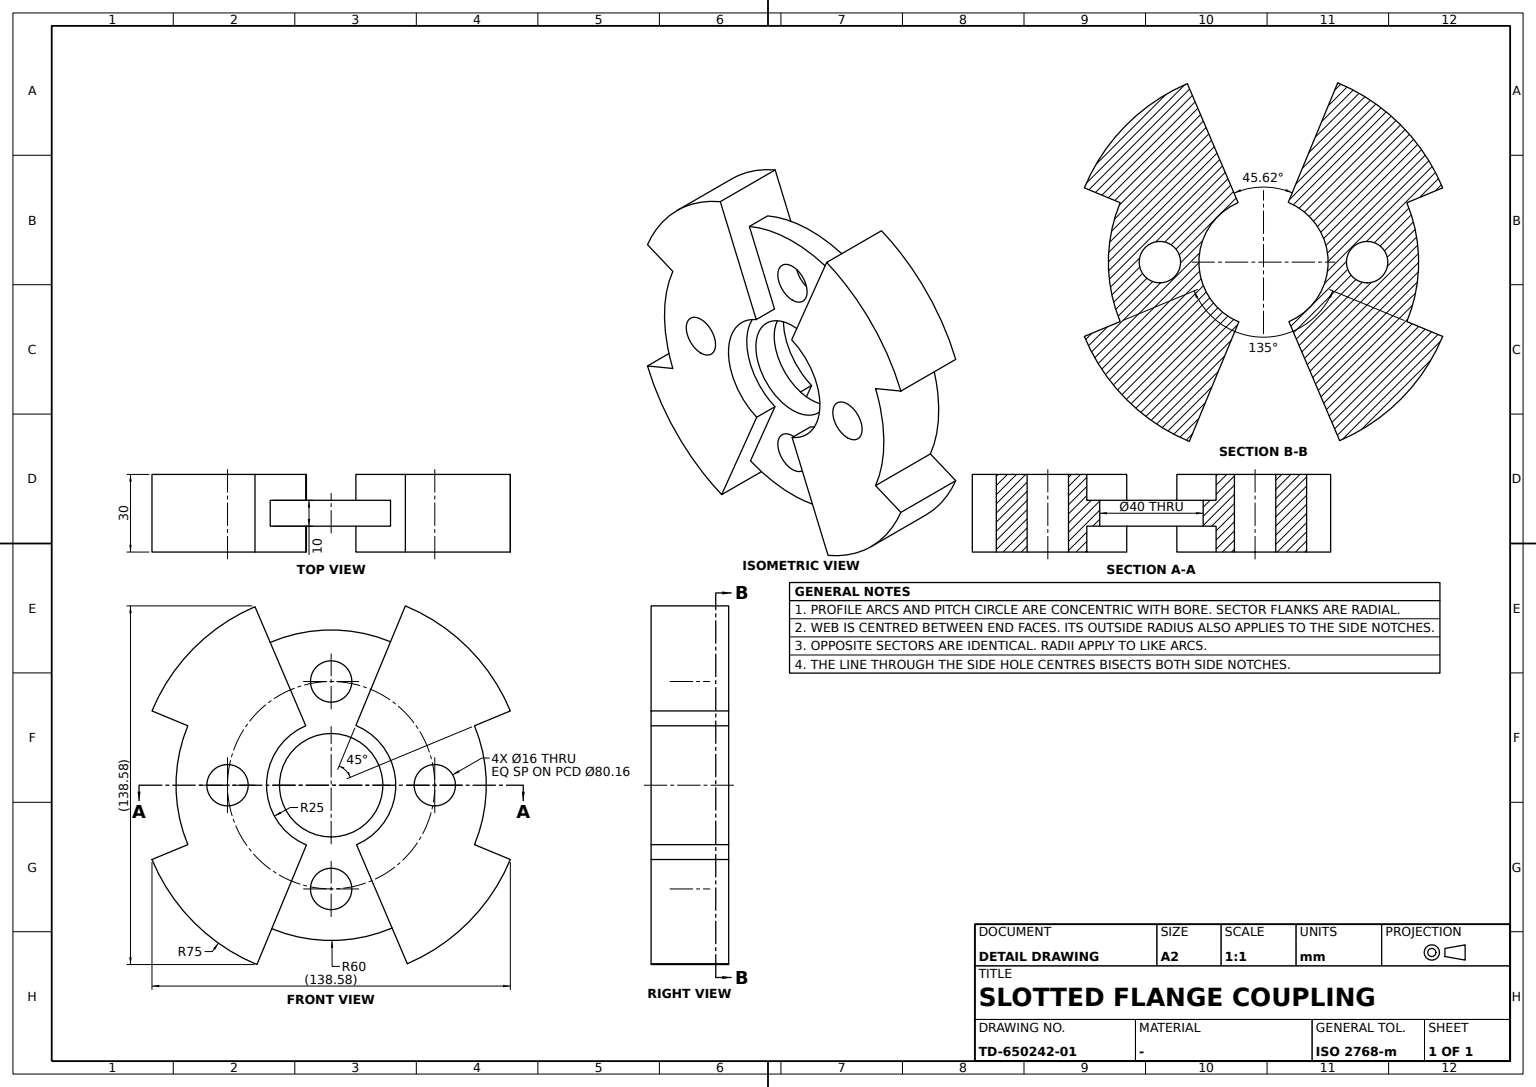
ISO-10303-21;
HEADER;
FILE_DESCRIPTION((''),'2;1');
FILE_NAME('','',(''),(''),'','','');
FILE_SCHEMA(('AUTOMOTIVE_DESIGN'));
ENDSEC;
DATA;
#1=APPLICATION_CONTEXT('');
#2=PRODUCT_CONTEXT('',#1,'mechanical');
#3=PRODUCT('','','',(#2));
#4=PRODUCT_DEFINITION_FORMATION('','',#3);
#5=PRODUCT_DEFINITION_CONTEXT('',#1,'design');
#6=PRODUCT_DEFINITION('','',#4,#5);
#7=PRODUCT_DEFINITION_SHAPE('','',#6);
#8=(LENGTH_UNIT()NAMED_UNIT(*)SI_UNIT(.MILLI.,.METRE.));
#9=(NAMED_UNIT(*)PLANE_ANGLE_UNIT()SI_UNIT($,.RADIAN.));
#10=(NAMED_UNIT(*)SI_UNIT($,.STERADIAN.)SOLID_ANGLE_UNIT());
#11=UNCERTAINTY_MEASURE_WITH_UNIT(LENGTH_MEASURE(0.005),#8,'distance_accuracy_value','');
#12=(GEOMETRIC_REPRESENTATION_CONTEXT(3)GLOBAL_UNCERTAINTY_ASSIGNED_CONTEXT((#11))GLOBAL_UNIT_ASSIGNED_CONTEXT((#8,#9,#10))REPRESENTATION_CONTEXT('',''));
#13=CARTESIAN_POINT('',(-5.,0.,-20.));
#14=VERTEX_POINT('',#13);
#15=CARTESIAN_POINT('',(-5.,0.,0.));
#16=DIRECTION('',(1.,0.,0.));
#17=DIRECTION('',(0.,0.,-1.));
#18=AXIS2_PLACEMENT_3D('',#15,#16,#17);
#19=CIRCLE('',#18,20.);
#20=EDGE_CURVE('',#14,#14,#19,.T.);
#21=ORIENTED_EDGE('',*,*,#20,.F.);
#22=EDGE_LOOP('',(#21));
#23=FACE_BOUND('',#22,.T.);
#24=CARTESIAN_POINT('',(5.,0.,-20.));
#25=VERTEX_POINT('',#24);
#26=CARTESIAN_POINT('',(5.,0.,0.));
#27=AXIS2_PLACEMENT_3D('',#26,#16,#17);
#28=CIRCLE('',#27,20.);
#29=EDGE_CURVE('',#25,#25,#28,.T.);
#30=ORIENTED_EDGE('',*,*,#29,.T.);
#31=EDGE_LOOP('',(#30));
#32=FACE_BOUND('',#31,.T.);
#33=CARTESIAN_POINT('',(0.,0.,0.));
#34=DIRECTION('',(0.,1.,0.));
#35=AXIS2_PLACEMENT_3D('',#33,#16,#34);
#36=CYLINDRICAL_SURFACE('',#35,20.);
#37=ADVANCED_FACE('',(#23,#32),#36,.F.);
#38=CARTESIAN_POINT('',(15.,-69.290965,-28.701257));
#39=VERTEX_POINT('',#38);
#40=CARTESIAN_POINT('',(15.,-28.701257,-69.290965));
#41=VERTEX_POINT('',#40);
#42=CARTESIAN_POINT('',(15.,0.,0.));
#43=AXIS2_PLACEMENT_3D('',#42,#16,#17);
#44=CIRCLE('',#43,75.);
#45=EDGE_CURVE('',#39,#41,#44,.T.);
#46=ORIENTED_EDGE('',*,*,#45,.F.);
#47=CARTESIAN_POINT('',(-15.,-69.290965,-28.701257));
#48=VERTEX_POINT('',#47);
#49=VECTOR('',#16,1000.);
#50=LINE('',#47,#49);
#51=EDGE_CURVE('',#48,#39,#50,.T.);
#52=ORIENTED_EDGE('',*,*,#51,.F.);
#53=CARTESIAN_POINT('',(-15.,-28.701257,-69.290965));
#54=VERTEX_POINT('',#53);
#55=CARTESIAN_POINT('',(-15.,0.,0.));
#56=AXIS2_PLACEMENT_3D('',#55,#16,#17);
#57=CIRCLE('',#56,75.);
#58=EDGE_CURVE('',#48,#54,#57,.T.);
#59=ORIENTED_EDGE('',*,*,#58,.T.);
#60=LINE('',#53,#49);
#61=EDGE_CURVE('',#54,#41,#60,.T.);
#62=ORIENTED_EDGE('',*,*,#61,.T.);
#63=EDGE_LOOP('',(#46,#52,#59,#62));
#64=FACE_BOUND('',#63,.T.);
#65=CYLINDRICAL_SURFACE('',#35,75.);
#66=ADVANCED_FACE('',(#64),#65,.T.);
#67=CARTESIAN_POINT('',(-15.,-55.432772,22.961006));
#68=VERTEX_POINT('',#67);
#69=CARTESIAN_POINT('',(-15.,-55.432772,-22.961006));
#70=VERTEX_POINT('',#69);
#71=CIRCLE('',#56,60.);
#72=EDGE_CURVE('',#68,#70,#71,.T.);
#73=ORIENTED_EDGE('',*,*,#72,.T.);
#74=CARTESIAN_POINT('',(15.,-55.432772,-22.961006));
#75=VERTEX_POINT('',#74);
#76=LINE('',#69,#49);
#77=EDGE_CURVE('',#70,#75,#76,.T.);
#78=ORIENTED_EDGE('',*,*,#77,.T.);
#79=CARTESIAN_POINT('',(15.,-55.432772,22.961006));
#80=VERTEX_POINT('',#79);
#81=CIRCLE('',#43,60.);
#82=EDGE_CURVE('',#80,#75,#81,.T.);
#83=ORIENTED_EDGE('',*,*,#82,.F.);
#84=LINE('',#67,#49);
#85=EDGE_CURVE('',#68,#80,#84,.T.);
#86=ORIENTED_EDGE('',*,*,#85,.F.);
#87=EDGE_LOOP('',(#73,#78,#83,#86));
#88=FACE_BOUND('',#87,.T.);
#89=CYLINDRICAL_SURFACE('',#35,60.);
#90=ADVANCED_FACE('',(#88),#89,.T.);
#91=CARTESIAN_POINT('',(-15.,-69.290965,28.701257));
#92=VERTEX_POINT('',#91);
#93=DIRECTION('',(0.,0.923879533,-0.382683432));
#94=VECTOR('',#93,1000.);
#95=LINE('',#55,#94);
#96=EDGE_CURVE('',#92,#68,#95,.T.);
#97=ORIENTED_EDGE('',*,*,#96,.T.);
#98=ORIENTED_EDGE('',*,*,#85,.T.);
#99=CARTESIAN_POINT('',(15.,-69.290965,28.701257));
#100=VERTEX_POINT('',#99);
#101=LINE('',#42,#94);
#102=EDGE_CURVE('',#100,#80,#101,.T.);
#103=ORIENTED_EDGE('',*,*,#102,.F.);
#104=LINE('',#91,#49);
#105=EDGE_CURVE('',#92,#100,#104,.T.);
#106=ORIENTED_EDGE('',*,*,#105,.F.);
#107=EDGE_LOOP('',(#97,#98,#103,#106));
#108=FACE_BOUND('',#107,.T.);
#109=CARTESIAN_POINT('',(0.,-69.290965,28.701257));
#110=DIRECTION('',(0.,-0.382683432,-0.923879533));
#111=AXIS2_PLACEMENT_3D('',#109,#110,#93);
#112=PLANE('',#111);
#113=ADVANCED_FACE('',(#108),#112,.T.);
#114=CARTESIAN_POINT('',(5.,-9.818454,22.991258));
#115=VERTEX_POINT('',#114);
#116=CARTESIAN_POINT('',(15.,-9.818454,22.991258));
#117=VERTEX_POINT('',#116);
#118=LINE('',#114,#49);
#119=EDGE_CURVE('',#115,#117,#118,.T.);
#120=ORIENTED_EDGE('',*,*,#119,.T.);
#121=CARTESIAN_POINT('',(15.,-9.567086,-23.096988));
#122=VERTEX_POINT('',#121);
#123=CIRCLE('',#43,25.);
#124=EDGE_CURVE('',#117,#122,#123,.T.);
#125=ORIENTED_EDGE('',*,*,#124,.T.);
#126=CARTESIAN_POINT('',(5.,-9.567086,-23.096988));
#127=VERTEX_POINT('',#126);
#128=LINE('',#126,#49);
#129=EDGE_CURVE('',#127,#122,#128,.T.);
#130=ORIENTED_EDGE('',*,*,#129,.F.);
#131=CIRCLE('',#27,25.);
#132=EDGE_CURVE('',#115,#127,#131,.T.);
#133=ORIENTED_EDGE('',*,*,#132,.F.);
#134=EDGE_LOOP('',(#120,#125,#130,#133));
#135=FACE_BOUND('',#134,.T.);
#136=CYLINDRICAL_SURFACE('',#35,25.);
#137=ADVANCED_FACE('',(#135),#136,.F.);
#138=CARTESIAN_POINT('',(-15.,55.432772,-22.961006));
#139=VERTEX_POINT('',#138);
#140=CARTESIAN_POINT('',(15.,55.432772,-22.961006));
#141=VERTEX_POINT('',#140);
#142=LINE('',#138,#49);
#143=EDGE_CURVE('',#139,#141,#142,.T.);
#144=ORIENTED_EDGE('',*,*,#143,.F.);
#145=CARTESIAN_POINT('',(-15.,55.432772,22.961006));
#146=VERTEX_POINT('',#145);
#147=EDGE_CURVE('',#139,#146,#71,.T.);
#148=ORIENTED_EDGE('',*,*,#147,.T.);
#149=CARTESIAN_POINT('',(15.,55.432772,22.961006));
#150=VERTEX_POINT('',#149);
#151=LINE('',#145,#49);
#152=EDGE_CURVE('',#146,#150,#151,.T.);
#153=ORIENTED_EDGE('',*,*,#152,.T.);
#154=EDGE_CURVE('',#141,#150,#81,.T.);
#155=ORIENTED_EDGE('',*,*,#154,.F.);
#156=EDGE_LOOP('',(#144,#148,#153,#155));
#157=FACE_BOUND('',#156,.T.);
#158=ADVANCED_FACE('',(#157),#89,.T.);
#159=CARTESIAN_POINT('',(15.,-40.077698,-8.));
#160=VERTEX_POINT('',#159);
#161=CARTESIAN_POINT('',(15.,-40.077698,0.));
#162=AXIS2_PLACEMENT_3D('',#161,#16,#17);
#163=CIRCLE('',#162,8.);
#164=EDGE_CURVE('',#160,#160,#163,.T.);
#165=ORIENTED_EDGE('',*,*,#164,.F.);
#166=EDGE_LOOP('',(#165));
#167=FACE_BOUND('',#166,.T.);
#168=DIRECTION('',(0.,0.382683432,0.923879533));
#169=VECTOR('',#168,1000.);
#170=LINE('',#42,#169);
#171=EDGE_CURVE('',#41,#122,#170,.T.);
#172=ORIENTED_EDGE('',*,*,#171,.T.);
#173=ORIENTED_EDGE('',*,*,#124,.F.);
#174=CARTESIAN_POINT('',(15.,-29.455362,68.973775));
#175=VERTEX_POINT('',#174);
#176=DIRECTION('',(0.,-0.392738156,0.919650336));
#177=VECTOR('',#176,1000.);
#178=LINE('',#42,#177);
#179=EDGE_CURVE('',#117,#175,#178,.T.);
#180=ORIENTED_EDGE('',*,*,#179,.T.);
#181=EDGE_CURVE('',#175,#100,#44,.T.);
#182=ORIENTED_EDGE('',*,*,#181,.T.);
#183=ORIENTED_EDGE('',*,*,#102,.T.);
#184=ORIENTED_EDGE('',*,*,#82,.T.);
#185=DIRECTION('',(0.,0.923879533,0.382683432));
#186=VECTOR('',#185,1000.);
#187=LINE('',#42,#186);
#188=EDGE_CURVE('',#39,#75,#187,.T.);
#189=ORIENTED_EDGE('',*,*,#188,.F.);
#190=ORIENTED_EDGE('',*,*,#45,.T.);
#191=EDGE_LOOP('',(#172,#173,#180,#182,#183,#184,#189,#190));
#192=FACE_BOUND('',#191,.T.);
#193=AXIS2_PLACEMENT_3D('',#42,#16,#34);
#194=PLANE('',#193);
#195=ADVANCED_FACE('',(#167,#192),#194,.T.);
#196=CARTESIAN_POINT('',(5.,9.567086,23.096988));
#197=VERTEX_POINT('',#196);
#198=CARTESIAN_POINT('',(15.,9.567086,23.096988));
#199=VERTEX_POINT('',#198);
#200=LINE('',#196,#49);
#201=EDGE_CURVE('',#197,#199,#200,.T.);
#202=ORIENTED_EDGE('',*,*,#201,.F.);
#203=CARTESIAN_POINT('',(5.,9.818454,-22.991258));
#204=VERTEX_POINT('',#203);
#205=EDGE_CURVE('',#204,#197,#131,.T.);
#206=ORIENTED_EDGE('',*,*,#205,.F.);
#207=CARTESIAN_POINT('',(15.,9.818454,-22.991258));
#208=VERTEX_POINT('',#207);
#209=LINE('',#203,#49);
#210=EDGE_CURVE('',#204,#208,#209,.T.);
#211=ORIENTED_EDGE('',*,*,#210,.T.);
#212=EDGE_CURVE('',#208,#199,#123,.T.);
#213=ORIENTED_EDGE('',*,*,#212,.T.);
#214=EDGE_LOOP('',(#202,#206,#211,#213));
#215=FACE_BOUND('',#214,.T.);
#216=ADVANCED_FACE('',(#215),#136,.F.);
#217=ORIENTED_EDGE('',*,*,#143,.T.);
#218=CARTESIAN_POINT('',(15.,69.290965,-28.701257));
#219=VERTEX_POINT('',#218);
#220=EDGE_CURVE('',#141,#219,#101,.T.);
#221=ORIENTED_EDGE('',*,*,#220,.T.);
#222=CARTESIAN_POINT('',(-15.,69.290965,-28.701257));
#223=VERTEX_POINT('',#222);
#224=LINE('',#222,#49);
#225=EDGE_CURVE('',#223,#219,#224,.T.);
#226=ORIENTED_EDGE('',*,*,#225,.F.);
#227=EDGE_CURVE('',#139,#223,#95,.T.);
#228=ORIENTED_EDGE('',*,*,#227,.F.);
#229=EDGE_LOOP('',(#217,#221,#226,#228));
#230=FACE_BOUND('',#229,.T.);
#231=ADVANCED_FACE('',(#230),#112,.F.);
#232=ORIENTED_EDGE('',*,*,#171,.F.);
#233=ORIENTED_EDGE('',*,*,#61,.F.);
#234=CARTESIAN_POINT('',(-15.,-9.567086,-23.096988));
#235=VERTEX_POINT('',#234);
#236=LINE('',#55,#169);
#237=EDGE_CURVE('',#54,#235,#236,.T.);
#238=ORIENTED_EDGE('',*,*,#237,.T.);
#239=CARTESIAN_POINT('',(-5.,-9.567086,-23.096988));
#240=VERTEX_POINT('',#239);
#241=LINE('',#234,#49);
#242=EDGE_CURVE('',#235,#240,#241,.T.);
#243=ORIENTED_EDGE('',*,*,#242,.T.);
#244=CARTESIAN_POINT('',(-5.,-22.961006,-55.432772));
#245=VERTEX_POINT('',#244);
#246=LINE('',#15,#169);
#247=EDGE_CURVE('',#245,#240,#246,.T.);
#248=ORIENTED_EDGE('',*,*,#247,.F.);
#249=CARTESIAN_POINT('',(5.,-22.961006,-55.432772));
#250=VERTEX_POINT('',#249);
#251=LINE('',#244,#49);
#252=EDGE_CURVE('',#245,#250,#251,.T.);
#253=ORIENTED_EDGE('',*,*,#252,.T.);
#254=LINE('',#26,#169);
#255=EDGE_CURVE('',#250,#127,#254,.T.);
#256=ORIENTED_EDGE('',*,*,#255,.T.);
#257=ORIENTED_EDGE('',*,*,#129,.T.);
#258=EDGE_LOOP('',(#232,#233,#238,#243,#248,#253,#256,#257));
#259=FACE_BOUND('',#258,.T.);
#260=CARTESIAN_POINT('',(0.,-28.701257,-69.290965));
#261=AXIS2_PLACEMENT_3D('',#260,#93,#168);
#262=PLANE('',#261);
#263=ADVANCED_FACE('',(#259),#262,.T.);
#264=CARTESIAN_POINT('',(-15.,9.567086,23.096988));
#265=VERTEX_POINT('',#264);
#266=CARTESIAN_POINT('',(-15.,28.701257,69.290965));
#267=VERTEX_POINT('',#266);
#268=EDGE_CURVE('',#265,#267,#236,.T.);
#269=ORIENTED_EDGE('',*,*,#268,.T.);
#270=CARTESIAN_POINT('',(-15.,69.290965,28.701257));
#271=VERTEX_POINT('',#270);
#272=EDGE_CURVE('',#271,#267,#57,.T.);
#273=ORIENTED_EDGE('',*,*,#272,.F.);
#274=LINE('',#55,#186);
#275=EDGE_CURVE('',#146,#271,#274,.T.);
#276=ORIENTED_EDGE('',*,*,#275,.F.);
#277=ORIENTED_EDGE('',*,*,#147,.F.);
#278=ORIENTED_EDGE('',*,*,#227,.T.);
#279=CARTESIAN_POINT('',(-15.,29.455362,-68.973775));
#280=VERTEX_POINT('',#279);
#281=EDGE_CURVE('',#280,#223,#57,.T.);
#282=ORIENTED_EDGE('',*,*,#281,.F.);
#283=CARTESIAN_POINT('',(-15.,9.818454,-22.991258));
#284=VERTEX_POINT('',#283);
#285=LINE('',#55,#177);
#286=EDGE_CURVE('',#280,#284,#285,.T.);
#287=ORIENTED_EDGE('',*,*,#286,.T.);
#288=CIRCLE('',#56,25.);
#289=EDGE_CURVE('',#284,#265,#288,.T.);
#290=ORIENTED_EDGE('',*,*,#289,.T.);
#291=EDGE_LOOP('',(#269,#273,#276,#277,#278,#282,#287,#290));
#292=FACE_BOUND('',#291,.T.);
#293=CARTESIAN_POINT('',(-15.,40.077698,-8.));
#294=VERTEX_POINT('',#293);
#295=CARTESIAN_POINT('',(-15.,40.077698,0.));
#296=AXIS2_PLACEMENT_3D('',#295,#16,#17);
#297=CIRCLE('',#296,8.);
#298=EDGE_CURVE('',#294,#294,#297,.T.);
#299=ORIENTED_EDGE('',*,*,#298,.T.);
#300=EDGE_LOOP('',(#299));
#301=FACE_BOUND('',#300,.T.);
#302=AXIS2_PLACEMENT_3D('',#55,#16,#34);
#303=PLANE('',#302);
#304=ADVANCED_FACE('',(#292,#301),#303,.F.);
#305=CARTESIAN_POINT('',(5.,0.,32.077698));
#306=VERTEX_POINT('',#305);
#307=CARTESIAN_POINT('',(5.,0.,40.077698));
#308=AXIS2_PLACEMENT_3D('',#307,#16,#17);
#309=CIRCLE('',#308,8.);
#310=EDGE_CURVE('',#306,#306,#309,.T.);
#311=ORIENTED_EDGE('',*,*,#310,.F.);
#312=EDGE_LOOP('',(#311));
#313=FACE_BOUND('',#312,.T.);
#314=CARTESIAN_POINT('',(5.,22.961006,55.432772));
#315=VERTEX_POINT('',#314);
#316=CARTESIAN_POINT('',(5.,-23.564289,55.17902));
#317=VERTEX_POINT('',#316);
#318=CIRCLE('',#27,60.);
#319=EDGE_CURVE('',#315,#317,#318,.T.);
#320=ORIENTED_EDGE('',*,*,#319,.T.);
#321=DIRECTION('',(0.,0.392738156,-0.919650336));
#322=VECTOR('',#321,1000.);
#323=LINE('',#114,#322);
#324=EDGE_CURVE('',#317,#115,#323,.T.);
#325=ORIENTED_EDGE('',*,*,#324,.T.);
#326=ORIENTED_EDGE('',*,*,#132,.T.);
#327=ORIENTED_EDGE('',*,*,#255,.F.);
#328=CARTESIAN_POINT('',(5.,23.564289,-55.17902));
#329=VERTEX_POINT('',#328);
#330=EDGE_CURVE('',#250,#329,#318,.T.);
#331=ORIENTED_EDGE('',*,*,#330,.T.);
#332=LINE('',#26,#177);
#333=EDGE_CURVE('',#329,#204,#332,.T.);
#334=ORIENTED_EDGE('',*,*,#333,.T.);
#335=ORIENTED_EDGE('',*,*,#205,.T.);
#336=CARTESIAN_POINT('',(5.,-28.701257,-69.290965));
#337=VECTOR('',#110,1000.);
#338=LINE('',#336,#337);
#339=EDGE_CURVE('',#315,#197,#338,.T.);
#340=ORIENTED_EDGE('',*,*,#339,.F.);
#341=EDGE_LOOP('',(#320,#325,#326,#327,#331,#334,#335,#340));
#342=FACE_BOUND('',#341,.T.);
#343=CARTESIAN_POINT('',(5.,0.,-48.077698));
#344=VERTEX_POINT('',#343);
#345=CARTESIAN_POINT('',(5.,0.,-40.077698));
#346=AXIS2_PLACEMENT_3D('',#345,#16,#17);
#347=CIRCLE('',#346,8.);
#348=EDGE_CURVE('',#344,#344,#347,.T.);
#349=ORIENTED_EDGE('',*,*,#348,.F.);
#350=EDGE_LOOP('',(#349));
#351=FACE_BOUND('',#350,.T.);
#352=ORIENTED_EDGE('',*,*,#29,.F.);
#353=EDGE_LOOP('',(#352));
#354=FACE_BOUND('',#353,.T.);
#355=AXIS2_PLACEMENT_3D('',#26,#16,#34);
#356=PLANE('',#355);
#357=ADVANCED_FACE('',(#313,#342,#351,#354),#356,.T.);
#358=EDGE_CURVE('',#48,#70,#274,.T.);
#359=ORIENTED_EDGE('',*,*,#358,.F.);
#360=ORIENTED_EDGE('',*,*,#51,.T.);
#361=ORIENTED_EDGE('',*,*,#188,.T.);
#362=ORIENTED_EDGE('',*,*,#77,.F.);
#363=EDGE_LOOP('',(#359,#360,#361,#362));
#364=FACE_BOUND('',#363,.T.);
#365=CARTESIAN_POINT('',(0.,-69.290965,-28.701257));
#366=DIRECTION('',(0.,0.382683432,-0.923879533));
#367=AXIS2_PLACEMENT_3D('',#365,#366,#185);
#368=PLANE('',#367);
#369=ADVANCED_FACE('',(#364),#368,.F.);
#370=CARTESIAN_POINT('',(-5.,23.564289,-55.17902));
#371=VERTEX_POINT('',#370);
#372=CIRCLE('',#18,60.);
#373=EDGE_CURVE('',#245,#371,#372,.T.);
#374=ORIENTED_EDGE('',*,*,#373,.T.);
#375=LINE('',#370,#49);
#376=EDGE_CURVE('',#371,#329,#375,.T.);
#377=ORIENTED_EDGE('',*,*,#376,.T.);
#378=ORIENTED_EDGE('',*,*,#330,.F.);
#379=ORIENTED_EDGE('',*,*,#252,.F.);
#380=EDGE_LOOP('',(#374,#377,#378,#379));
#381=FACE_BOUND('',#380,.T.);
#382=ADVANCED_FACE('',(#381),#89,.T.);
#383=ORIENTED_EDGE('',*,*,#310,.T.);
#384=EDGE_LOOP('',(#383));
#385=FACE_BOUND('',#384,.T.);
#386=CARTESIAN_POINT('',(-5.,0.,32.077698));
#387=VERTEX_POINT('',#386);
#388=CARTESIAN_POINT('',(-5.,0.,40.077698));
#389=AXIS2_PLACEMENT_3D('',#388,#16,#17);
#390=CIRCLE('',#389,8.);
#391=EDGE_CURVE('',#387,#387,#390,.T.);
#392=ORIENTED_EDGE('',*,*,#391,.F.);
#393=EDGE_LOOP('',(#392));
#394=FACE_BOUND('',#393,.T.);
#395=CARTESIAN_POINT('',(0.,0.,40.077698));
#396=AXIS2_PLACEMENT_3D('',#395,#16,#34);
#397=CYLINDRICAL_SURFACE('',#396,8.);
#398=ADVANCED_FACE('',(#385,#394),#397,.F.);
#399=CARTESIAN_POINT('',(-5.,22.961006,55.432772));
#400=VERTEX_POINT('',#399);
#401=CARTESIAN_POINT('',(-5.,-23.564289,55.17902));
#402=VERTEX_POINT('',#401);
#403=EDGE_CURVE('',#400,#402,#372,.T.);
#404=ORIENTED_EDGE('',*,*,#403,.T.);
#405=LINE('',#401,#49);
#406=EDGE_CURVE('',#402,#317,#405,.T.);
#407=ORIENTED_EDGE('',*,*,#406,.T.);
#408=ORIENTED_EDGE('',*,*,#319,.F.);
#409=LINE('',#399,#49);
#410=EDGE_CURVE('',#400,#315,#409,.T.);
#411=ORIENTED_EDGE('',*,*,#410,.F.);
#412=EDGE_LOOP('',(#404,#407,#408,#411));
#413=FACE_BOUND('',#412,.T.);
#414=ADVANCED_FACE('',(#413),#89,.T.);
#415=CARTESIAN_POINT('',(-5.,-9.818454,22.991258));
#416=VERTEX_POINT('',#415);
#417=LINE('',#415,#322);
#418=EDGE_CURVE('',#402,#416,#417,.T.);
#419=ORIENTED_EDGE('',*,*,#418,.T.);
#420=CARTESIAN_POINT('',(-15.,-9.818454,22.991258));
#421=VERTEX_POINT('',#420);
#422=LINE('',#420,#49);
#423=EDGE_CURVE('',#421,#416,#422,.T.);
#424=ORIENTED_EDGE('',*,*,#423,.F.);
#425=CARTESIAN_POINT('',(-15.,-29.455362,68.973775));
#426=VERTEX_POINT('',#425);
#427=EDGE_CURVE('',#421,#426,#285,.T.);
#428=ORIENTED_EDGE('',*,*,#427,.T.);
#429=LINE('',#425,#49);
#430=EDGE_CURVE('',#426,#175,#429,.T.);
#431=ORIENTED_EDGE('',*,*,#430,.T.);
#432=ORIENTED_EDGE('',*,*,#179,.F.);
#433=ORIENTED_EDGE('',*,*,#119,.F.);
#434=ORIENTED_EDGE('',*,*,#324,.F.);
#435=ORIENTED_EDGE('',*,*,#406,.F.);
#436=EDGE_LOOP('',(#419,#424,#428,#431,#432,#433,#434,#435));
#437=FACE_BOUND('',#436,.T.);
#438=CARTESIAN_POINT('',(0.,-9.818454,22.991258));
#439=DIRECTION('',(0.,0.919650336,0.392738156));
#440=AXIS2_PLACEMENT_3D('',#438,#439,#176);
#441=PLANE('',#440);
#442=ADVANCED_FACE('',(#437),#441,.T.);
#443=CARTESIAN_POINT('',(15.,28.701257,69.290965));
#444=VERTEX_POINT('',#443);
#445=EDGE_CURVE('',#199,#444,#170,.T.);
#446=ORIENTED_EDGE('',*,*,#445,.T.);
#447=LINE('',#266,#49);
#448=EDGE_CURVE('',#267,#444,#447,.T.);
#449=ORIENTED_EDGE('',*,*,#448,.F.);
#450=ORIENTED_EDGE('',*,*,#268,.F.);
#451=CARTESIAN_POINT('',(-5.,9.567086,23.096988));
#452=VERTEX_POINT('',#451);
#453=LINE('',#264,#49);
#454=EDGE_CURVE('',#265,#452,#453,.T.);
#455=ORIENTED_EDGE('',*,*,#454,.T.);
#456=CARTESIAN_POINT('',(-5.,-28.701257,-69.290965));
#457=LINE('',#456,#337);
#458=EDGE_CURVE('',#400,#452,#457,.T.);
#459=ORIENTED_EDGE('',*,*,#458,.F.);
#460=ORIENTED_EDGE('',*,*,#410,.T.);
#461=ORIENTED_EDGE('',*,*,#339,.T.);
#462=ORIENTED_EDGE('',*,*,#201,.T.);
#463=EDGE_LOOP('',(#446,#449,#450,#455,#459,#460,#461,#462));
#464=FACE_BOUND('',#463,.T.);
#465=ADVANCED_FACE('',(#464),#262,.F.);
#466=ORIENTED_EDGE('',*,*,#242,.F.);
#467=EDGE_CURVE('',#421,#235,#288,.T.);
#468=ORIENTED_EDGE('',*,*,#467,.F.);
#469=ORIENTED_EDGE('',*,*,#423,.T.);
#470=CIRCLE('',#18,25.);
#471=EDGE_CURVE('',#416,#240,#470,.T.);
#472=ORIENTED_EDGE('',*,*,#471,.T.);
#473=EDGE_LOOP('',(#466,#468,#469,#472));
#474=FACE_BOUND('',#473,.T.);
#475=ADVANCED_FACE('',(#474),#136,.F.);
#476=CARTESIAN_POINT('',(15.,29.455362,-68.973775));
#477=VERTEX_POINT('',#476);
#478=EDGE_CURVE('',#477,#219,#44,.T.);
#479=ORIENTED_EDGE('',*,*,#478,.F.);
#480=LINE('',#279,#49);
#481=EDGE_CURVE('',#280,#477,#480,.T.);
#482=ORIENTED_EDGE('',*,*,#481,.F.);
#483=ORIENTED_EDGE('',*,*,#281,.T.);
#484=ORIENTED_EDGE('',*,*,#225,.T.);
#485=EDGE_LOOP('',(#479,#482,#483,#484));
#486=FACE_BOUND('',#485,.T.);
#487=ADVANCED_FACE('',(#486),#65,.T.);
#488=ORIENTED_EDGE('',*,*,#391,.T.);
#489=EDGE_LOOP('',(#488));
#490=FACE_BOUND('',#489,.T.);
#491=ORIENTED_EDGE('',*,*,#20,.T.);
#492=EDGE_LOOP('',(#491));
#493=FACE_BOUND('',#492,.T.);
#494=ORIENTED_EDGE('',*,*,#247,.T.);
#495=ORIENTED_EDGE('',*,*,#471,.F.);
#496=ORIENTED_EDGE('',*,*,#418,.F.);
#497=ORIENTED_EDGE('',*,*,#403,.F.);
#498=ORIENTED_EDGE('',*,*,#458,.T.);
#499=CARTESIAN_POINT('',(-5.,9.818454,-22.991258));
#500=VERTEX_POINT('',#499);
#501=EDGE_CURVE('',#500,#452,#470,.T.);
#502=ORIENTED_EDGE('',*,*,#501,.F.);
#503=LINE('',#15,#177);
#504=EDGE_CURVE('',#371,#500,#503,.T.);
#505=ORIENTED_EDGE('',*,*,#504,.F.);
#506=ORIENTED_EDGE('',*,*,#373,.F.);
#507=EDGE_LOOP('',(#494,#495,#496,#497,#498,#502,#505,#506));
#508=FACE_BOUND('',#507,.T.);
#509=CARTESIAN_POINT('',(-5.,0.,-48.077698));
#510=VERTEX_POINT('',#509);
#511=CARTESIAN_POINT('',(-5.,0.,-40.077698));
#512=AXIS2_PLACEMENT_3D('',#511,#16,#17);
#513=CIRCLE('',#512,8.);
#514=EDGE_CURVE('',#510,#510,#513,.T.);
#515=ORIENTED_EDGE('',*,*,#514,.T.);
#516=EDGE_LOOP('',(#515));
#517=FACE_BOUND('',#516,.T.);
#518=AXIS2_PLACEMENT_3D('',#15,#16,#34);
#519=PLANE('',#518);
#520=ADVANCED_FACE('',(#490,#493,#508,#517),#519,.F.);
#521=CARTESIAN_POINT('',(15.,40.077698,-8.));
#522=VERTEX_POINT('',#521);
#523=CARTESIAN_POINT('',(15.,40.077698,0.));
#524=AXIS2_PLACEMENT_3D('',#523,#16,#17);
#525=CIRCLE('',#524,8.);
#526=EDGE_CURVE('',#522,#522,#525,.T.);
#527=ORIENTED_EDGE('',*,*,#526,.T.);
#528=EDGE_LOOP('',(#527));
#529=FACE_BOUND('',#528,.T.);
#530=ORIENTED_EDGE('',*,*,#298,.F.);
#531=EDGE_LOOP('',(#530));
#532=FACE_BOUND('',#531,.T.);
#533=CARTESIAN_POINT('',(0.,40.077698,0.));
#534=AXIS2_PLACEMENT_3D('',#533,#16,#34);
#535=CYLINDRICAL_SURFACE('',#534,8.);
#536=ADVANCED_FACE('',(#529,#532),#535,.F.);
#537=CARTESIAN_POINT('',(15.,69.290965,28.701257));
#538=VERTEX_POINT('',#537);
#539=LINE('',#270,#49);
#540=EDGE_CURVE('',#271,#538,#539,.T.);
#541=ORIENTED_EDGE('',*,*,#540,.T.);
#542=EDGE_CURVE('',#150,#538,#187,.T.);
#543=ORIENTED_EDGE('',*,*,#542,.F.);
#544=ORIENTED_EDGE('',*,*,#152,.F.);
#545=ORIENTED_EDGE('',*,*,#275,.T.);
#546=EDGE_LOOP('',(#541,#543,#544,#545));
#547=FACE_BOUND('',#546,.T.);
#548=ADVANCED_FACE('',(#547),#368,.T.);
#549=ORIENTED_EDGE('',*,*,#348,.T.);
#550=EDGE_LOOP('',(#549));
#551=FACE_BOUND('',#550,.T.);
#552=ORIENTED_EDGE('',*,*,#514,.F.);
#553=EDGE_LOOP('',(#552));
#554=FACE_BOUND('',#553,.T.);
#555=CARTESIAN_POINT('',(0.,0.,-40.077698));
#556=AXIS2_PLACEMENT_3D('',#555,#16,#34);
#557=CYLINDRICAL_SURFACE('',#556,8.);
#558=ADVANCED_FACE('',(#551,#554),#557,.F.);
#559=ORIENTED_EDGE('',*,*,#448,.T.);
#560=EDGE_CURVE('',#538,#444,#44,.T.);
#561=ORIENTED_EDGE('',*,*,#560,.F.);
#562=ORIENTED_EDGE('',*,*,#540,.F.);
#563=ORIENTED_EDGE('',*,*,#272,.T.);
#564=EDGE_LOOP('',(#559,#561,#562,#563));
#565=FACE_BOUND('',#564,.T.);
#566=ADVANCED_FACE('',(#565),#65,.T.);
#567=ORIENTED_EDGE('',*,*,#181,.F.);
#568=ORIENTED_EDGE('',*,*,#430,.F.);
#569=EDGE_CURVE('',#426,#92,#57,.T.);
#570=ORIENTED_EDGE('',*,*,#569,.T.);
#571=ORIENTED_EDGE('',*,*,#105,.T.);
#572=EDGE_LOOP('',(#567,#568,#570,#571));
#573=FACE_BOUND('',#572,.T.);
#574=ADVANCED_FACE('',(#573),#65,.T.);
#575=ORIENTED_EDGE('',*,*,#445,.F.);
#576=ORIENTED_EDGE('',*,*,#212,.F.);
#577=EDGE_CURVE('',#477,#208,#178,.T.);
#578=ORIENTED_EDGE('',*,*,#577,.F.);
#579=ORIENTED_EDGE('',*,*,#478,.T.);
#580=ORIENTED_EDGE('',*,*,#220,.F.);
#581=ORIENTED_EDGE('',*,*,#154,.T.);
#582=ORIENTED_EDGE('',*,*,#542,.T.);
#583=ORIENTED_EDGE('',*,*,#560,.T.);
#584=EDGE_LOOP('',(#575,#576,#578,#579,#580,#581,#582,#583));
#585=FACE_BOUND('',#584,.T.);
#586=ORIENTED_EDGE('',*,*,#526,.F.);
#587=EDGE_LOOP('',(#586));
#588=FACE_BOUND('',#587,.T.);
#589=ADVANCED_FACE('',(#585,#588),#194,.T.);
#590=ORIENTED_EDGE('',*,*,#376,.F.);
#591=ORIENTED_EDGE('',*,*,#504,.T.);
#592=LINE('',#283,#49);
#593=EDGE_CURVE('',#284,#500,#592,.T.);
#594=ORIENTED_EDGE('',*,*,#593,.F.);
#595=ORIENTED_EDGE('',*,*,#286,.F.);
#596=ORIENTED_EDGE('',*,*,#481,.T.);
#597=ORIENTED_EDGE('',*,*,#577,.T.);
#598=ORIENTED_EDGE('',*,*,#210,.F.);
#599=ORIENTED_EDGE('',*,*,#333,.F.);
#600=EDGE_LOOP('',(#590,#591,#594,#595,#596,#597,#598,#599));
#601=FACE_BOUND('',#600,.T.);
#602=ADVANCED_FACE('',(#601),#441,.F.);
#603=ORIENTED_EDGE('',*,*,#164,.T.);
#604=EDGE_LOOP('',(#603));
#605=FACE_BOUND('',#604,.T.);
#606=CARTESIAN_POINT('',(-15.,-40.077698,-8.));
#607=VERTEX_POINT('',#606);
#608=CARTESIAN_POINT('',(-15.,-40.077698,0.));
#609=AXIS2_PLACEMENT_3D('',#608,#16,#17);
#610=CIRCLE('',#609,8.);
#611=EDGE_CURVE('',#607,#607,#610,.T.);
#612=ORIENTED_EDGE('',*,*,#611,.F.);
#613=EDGE_LOOP('',(#612));
#614=FACE_BOUND('',#613,.T.);
#615=CARTESIAN_POINT('',(0.,-40.077698,0.));
#616=AXIS2_PLACEMENT_3D('',#615,#16,#34);
#617=CYLINDRICAL_SURFACE('',#616,8.);
#618=ADVANCED_FACE('',(#605,#614),#617,.F.);
#619=ORIENTED_EDGE('',*,*,#501,.T.);
#620=ORIENTED_EDGE('',*,*,#454,.F.);
#621=ORIENTED_EDGE('',*,*,#289,.F.);
#622=ORIENTED_EDGE('',*,*,#593,.T.);
#623=EDGE_LOOP('',(#619,#620,#621,#622));
#624=FACE_BOUND('',#623,.T.);
#625=ADVANCED_FACE('',(#624),#136,.F.);
#626=ORIENTED_EDGE('',*,*,#611,.T.);
#627=EDGE_LOOP('',(#626));
#628=FACE_BOUND('',#627,.T.);
#629=ORIENTED_EDGE('',*,*,#96,.F.);
#630=ORIENTED_EDGE('',*,*,#569,.F.);
#631=ORIENTED_EDGE('',*,*,#427,.F.);
#632=ORIENTED_EDGE('',*,*,#467,.T.);
#633=ORIENTED_EDGE('',*,*,#237,.F.);
#634=ORIENTED_EDGE('',*,*,#58,.F.);
#635=ORIENTED_EDGE('',*,*,#358,.T.);
#636=ORIENTED_EDGE('',*,*,#72,.F.);
#637=EDGE_LOOP('',(#629,#630,#631,#632,#633,#634,#635,#636));
#638=FACE_BOUND('',#637,.T.);
#639=ADVANCED_FACE('',(#628,#638),#303,.F.);
#640=CLOSED_SHELL('',(#37,#66,#90,#113,#137,#158,#195,#216,#231,#263,#304,#357,#369,#382,#398,#414,#442,#465,#475,#487,#520,#536,#548,#558,#566,#574,#589,#602,#618,#625,#639));
#641=MANIFOLD_SOLID_BREP('',#640);
#642=ADVANCED_BREP_SHAPE_REPRESENTATION('',(#641),#12);
#643=SHAPE_DEFINITION_REPRESENTATION(#7,#642);
ENDSEC;
END-ISO-10303-21;
